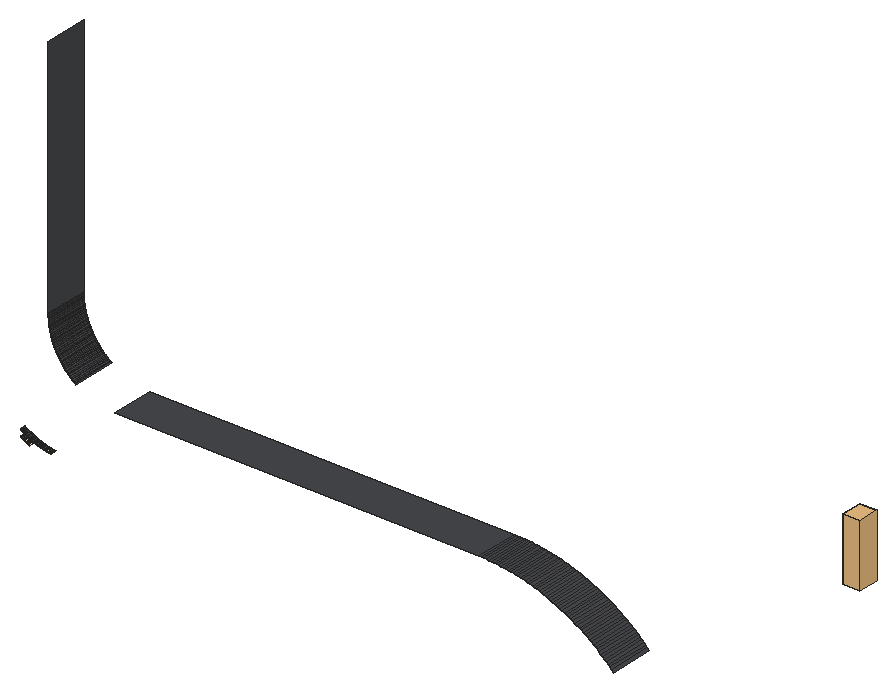
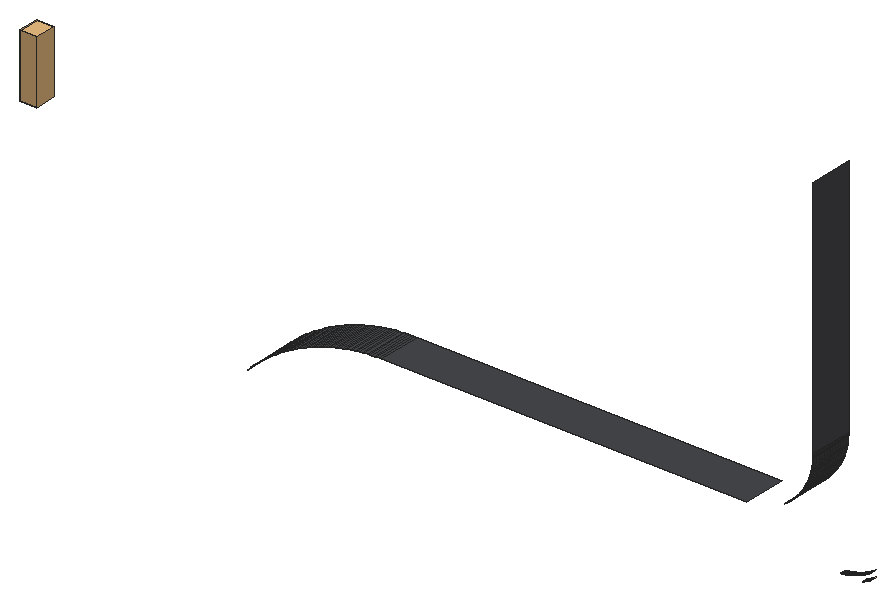
# SketchUp Ruby script. Lengths in inches.
U = 1.inch
M = Sketchup.active_model
def pt(a) = Geom::Point3d.new(a.map { |v| v * U })
def face(e, loops, mat)
  f = e.add_face(loops[0].map { |a| pt(a) })
  loops[1..].each { |l| e.add_face(l.map { |a| pt(a) }).erase! }
  f.material = f.back_material = mat if mat
  f
end
# faces: each face lists its corners as indices into pts; further lists are holes
def faces(e, pts, list, mat = nil) = list.each { |f| face(e, (f[0].is_a?(Array) ? f : [f]).map { |l| l.map { |i| pts[i] } }, mat) }
# xy, xz, yz: faces in a plane at the given z, y or x. An outline is a flat list of corners, or four numbers for a rectangle; further outlines are holes
def ring(l) = l.size == 4 ? [[l[0], l[1]], [l[2], l[1]], [l[2], l[3]], [l[0], l[3]]] : l.each_slice(2).to_a
def flat(e, list, mat, &to3) = list.each { |f| face(e, (f[0].is_a?(Array) ? f : [f]).map { |l| ring(l).map { |u, v| to3.(u, v) } }, mat) }
def xy(e, z, list, mat = nil) = flat(e, list, mat) { |x, y| [x, y, z] }
def xz(e, y, list, mat = nil) = flat(e, list, mat) { |x, z| [x, y, z] }
def yz(e, x, list, mat = nil) = flat(e, list, mat) { |y, z| [x, y, z] }
def lines(e, pts, list) = list.each { |a, b| e.add_line(pt(pts[a]), pt(pts[b])) }
# prism: a flat outline (further loops are holes) pulled along v
def prism(e, loops, v, mat = nil)
  f = face(e, loops, mat); d = Geom::Vector3d.new(v.map { |x| x * U })
  f.pushpull(f.normal.samedirection?(d) ? d.length : -d.length)
end
def box(e, o, s, mat = nil) = prism(e, [[o, [o[0] + s[0], o[1], o[2]], [o[0] + s[0], o[1] + s[1], o[2]], [o[0], o[1] + s[1], o[2]]]], [0, 0, s[2]], mat)
def at(x, y, z, deg = 0) = Geom::Transformation.translation(pt([x, y, z])) * Geom::Transformation.rotation(ORIGIN, Z_AXIS, deg.degrees)
def axes(o, x, y, z) = Geom::Transformation.new([*x, 0, *y, 0, *z, 0, *pt(o).to_a, 1])
def part(name) = M.definitions.add(name)
# library, detail: a bought-in or finely detailed component or shape, given as its bounding box
def library(name, o, s) = part(name).tap { |d| box(d.entities, o, s) }
def detail(e, o, s) = box(e.add_group.entities, o, s)
def put(e, d, t, mat = nil) = e.add_instance(d, t).tap { |i| i.material = mat if mat }
def group(e, t, mat = nil) = e.add_group.tap { |g| g.transformation = t; g.material = mat if mat }.entities
root = M.entities
M.materials.add("1432 AP 8245 TAR ROAD").color = [71, 72, 75]
M.materials.add("Outer Light").color = [251, 217, 152]
c1 = library("WALL LIGHT 69",[4.19,4.05,-8.78],[4.61,5.7,17.13])
xy(root,461.79,[[294,95.37,393,107.37],[393,95.37,393.67,107.37]],"1432 AP 8245 TAR ROAD")
yz(root,276,[[95.37,479.56,107.37,479.79],[95.37,479.79,107.37,545.79]],"1432 AP 8245 TAR ROAD")
yz(root,276.01,[[95.37,479.09,107.37,479.32]],"1432 AP 8245 TAR ROAD")
p = [[270.86,96.87,445.98],[271.01,96.87,445.91],[271.01,95.37,445.91],[270.86,95.37,445.98],[270.86,95.37,445.98],[271.01,95.37,445.91],
  [271.01,96.87,445.91],[270.86,96.87,445.98],[276.62,95.37,445.94],[276.47,95.37,445.96],[276.47,96.87,445.96],[276.62,96.87,445.94],
  [276.62,96.87,445.94],[276.47,96.87,445.96],[276.47,95.37,445.96],[276.62,95.37,445.94],[276.77,95.37,445.92],[276.77,96.87,445.92],
  [276.77,96.87,445.92],[276.77,95.37,445.92],[276.92,95.37,445.91],[276.92,96.87,445.91],[276.92,96.87,445.91],[276.92,95.37,445.91],
  [270.5625,96.87,446.11],[270.71,96.87,446.04],[270.71,95.37,446.04],[270.5625,95.37,446.11],[270.5625,95.37,446.11],[270.71,95.37,446.04],
  [270.71,96.87,446.04],[270.5625,96.87,446.11],[275.88,95.37,446.05],[275.73,95.37,446.07],[275.73,96.87,446.07],[275.88,96.87,446.05],
  [275.88,96.87,446.05],[275.73,96.87,446.07],[275.73,95.37,446.07],[275.88,95.37,446.05],[276.03,95.37,446.03],[276.03,96.87,446.03],
  [276.03,96.87,446.03],[276.03,95.37,446.03],[276.18,95.37,446],[276.18,96.87,446],[276.18,96.87,446],[276.18,95.37,446],
  [276.32,95.37,445.98],[276.32,96.87,445.98],[276.32,96.87,445.98],[276.32,95.37,445.98],[270.42,96.87,446.18],[270.42,95.37,446.18],
  [270.42,95.37,446.18],[270.42,96.87,446.18],[275.44,95.37,446.13],[275.29,95.37,446.16],[275.29,96.87,446.16],[275.44,96.87,446.13],
  [275.44,96.87,446.13],[275.29,96.87,446.16],[275.29,95.37,446.16],[275.44,95.37,446.13],[275.59,95.37,446.1],[275.59,96.87,446.1],
  [275.59,96.87,446.1],[275.59,95.37,446.1],[270.125,96.87,446.3125],[270.27,96.87,446.24],[270.27,95.37,446.24],[270.125,95.37,446.3125],
  [270.125,95.37,446.3125],[270.27,95.37,446.24],[270.27,96.87,446.24],[270.125,96.87,446.3125],[274.86,95.37,446.25],[274.71,95.37,446.28],
  [274.71,96.87,446.28],[274.86,96.87,446.25],[274.86,96.87,446.25],[274.71,96.87,446.28],[274.71,95.37,446.28],[274.86,95.37,446.25],
  [275,95.37,446.22],[275,96.87,446.22],[275,96.87,446.22],[275,95.37,446.22],[275.15,95.37,446.1875],[275.15,96.87,446.1875],
  [275.15,96.87,446.1875],[275.15,95.37,446.1875],[269.98,96.87,446.38],[269.98,95.37,446.38],[269.98,95.37,446.38],[269.98,96.87,446.38],
  [274.56,95.37,446.32],[274.42,95.37,446.35],[274.42,96.87,446.35],[274.56,96.87,446.32],[274.56,96.87,446.32],[274.42,96.87,446.35],
  [274.42,95.37,446.35],[274.56,95.37,446.32],[269.84,96.87,446.45],[269.84,95.37,446.45],[269.84,95.37,446.45],[269.84,96.87,446.45],
  [274.13,95.37,446.43],[273.99,95.37,446.47],[273.99,96.87,446.47],[274.13,96.87,446.43],[274.13,96.87,446.43],[273.99,96.87,446.47],
  [273.99,95.37,446.47],[274.13,95.37,446.43],[274.27,95.37,446.39],[274.27,96.87,446.39],[274.27,96.87,446.39],[274.27,95.37,446.39],
  [429.53,107.37,446.38],[429.0625,107.37,446.85],[429.0625,95.37,446.85],[429.53,95.37,446.38],[269.55,96.87,446.6],[269.69,96.87,446.53],
  [269.69,95.37,446.53],[269.55,95.37,446.6],[269.55,95.37,446.6],[269.69,95.37,446.53],[269.69,96.87,446.53],[269.55,96.87,446.6],
  [273.7,95.37,446.55],[273.56,95.37,446.59],[273.56,96.87,446.59],[273.7,96.87,446.55],[273.7,96.87,446.55],[273.56,96.87,446.59],
  [273.56,95.37,446.59],[273.7,95.37,446.55],[273.84,95.37,446.51],[273.84,96.87,446.51],[273.84,96.87,446.51],[273.84,95.37,446.51],
  [269.41,96.87,446.67],[269.41,95.37,446.67],[269.41,95.37,446.67],[269.41,96.87,446.67],[273.41,95.37,446.63],[273.27,95.37,446.68],
  [273.27,96.87,446.68],[273.41,96.87,446.63],[273.41,96.87,446.63],[273.27,96.87,446.68],[273.27,95.37,446.68],[273.41,95.37,446.63],
  [269.27,96.87,446.75],[269.27,95.37,446.75],[269.27,95.37,446.75],[269.27,96.87,446.75],[273.13,95.37,446.72],[272.99,95.37,446.77],
  [272.99,96.87,446.77],[273.13,96.87,446.72],[273.13,96.87,446.72],[272.99,96.87,446.77],[272.99,95.37,446.77],[273.13,95.37,446.72],
  [268.98,96.87,446.91],[269.125,96.87,446.83],[269.125,95.37,446.83],[268.98,95.37,446.91],[268.98,95.37,446.91],[269.125,95.37,446.83],
  [269.125,96.87,446.83],[268.98,96.87,446.91],[272.85,95.37,446.82],[272.7,95.37,446.87],[272.7,96.87,446.87],[272.85,96.87,446.82],
  [272.85,96.87,446.82],[272.7,96.87,446.87],[272.7,95.37,446.87],[272.85,95.37,446.82],[268.84,96.87,446.99],[268.84,95.37,446.99],
  [268.84,95.37,446.99],[268.84,96.87,446.99],[272.5625,95.37,446.92],[272.42,95.37,446.97],[272.42,96.87,446.97],[272.5625,96.87,446.92],
  [272.5625,96.87,446.92],[272.42,96.87,446.97],[272.42,95.37,446.97],[272.5625,95.37,446.92],[428.59,107.37,447.32],[428.59,95.37,447.32],
  [268.7,96.87,447.07],[268.7,95.37,447.07],[268.7,95.37,447.07],[268.7,96.87,447.07],[272.28,95.37,447.02],[272.14,95.37,447.07],
  [272.14,96.87,447.07],[272.28,96.87,447.02],[272.28,96.87,447.02],[272.14,96.87,447.07],[272.14,95.37,447.07],[272.28,95.37,447.02],
  [268.43,96.87,447.23],[268.56,96.87,447.15],[268.56,95.37,447.15],[268.43,95.37,447.23],[268.56,95.37,447.15],[268.56,96.87,447.15],
  [272.01,95.37,447.125],[271.87,95.37,447.18],[271.87,96.87,447.18],[272.01,96.87,447.125],[272.01,96.87,447.125],[271.87,96.87,447.18],
  [271.87,95.37,447.18],[272.01,95.37,447.125],[271.73,95.37,447.24],[271.59,95.37,447.3],[271.59,96.87,447.3],[271.73,96.87,447.24],
  [271.73,96.87,447.24],[271.59,96.87,447.3],[271.59,95.37,447.3],[271.73,95.37,447.24],[271.45,95.37,447.35],[271.45,96.87,447.35],
  [271.45,96.87,447.35],[271.45,95.37,447.35],[428.11,107.37,447.79],[428.11,95.37,447.79],[271.32,95.37,447.41],[271.18,95.37,447.48],
  [271.18,96.87,447.48],[271.32,96.87,447.41],[271.32,96.87,447.41],[271.18,96.87,447.48],[271.18,95.37,447.48],[271.32,95.37,447.41],
  [271.05,95.37,447.54],[270.91,95.37,447.6],[270.91,96.87,447.6],[271.05,96.87,447.54],[271.05,96.87,447.54],[270.91,96.87,447.6],
  [270.91,95.37,447.6],[271.05,95.37,447.54],[270.78,95.37,447.66],[270.78,96.87,447.66],[270.78,96.87,447.66],[270.78,95.37,447.66],
  [270.64,95.37,447.73],[270.51,95.37,447.8],[270.51,96.87,447.8],[270.64,96.87,447.73],[270.64,96.87,447.73],[270.51,96.87,447.8],
  [270.51,95.37,447.8],[270.64,95.37,447.73],[270.375,95.37,447.86],[270.375,96.87,447.86],[270.375,96.87,447.86],[270.375,95.37,447.86],
  [427.62,107.37,448.24],[427.62,95.37,448.24],[270.24,95.37,447.93],[270.11,95.37,448],[270.11,96.87,448],[270.24,96.87,447.93],
  [270.24,96.87,447.93],[270.11,96.87,448],[270.11,95.37,448],[270.24,95.37,447.93],[269.98,95.37,448.07],[269.98,96.87,448.07],
  [269.98,96.87,448.07],[269.98,95.37,448.07],[269.85,95.37,448.14],[269.72,95.37,448.21],[269.72,96.87,448.21],[269.85,96.87,448.14],
  [269.85,96.87,448.14],[269.72,96.87,448.21],[269.72,95.37,448.21],[269.85,95.37,448.14],[269.59,95.37,448.29],[269.59,96.87,448.29],
  [269.59,96.87,448.29],[269.59,95.37,448.29],[427.125,107.37,448.69],[427.125,95.37,448.69],[269.46,95.37,448.36],[269.46,96.87,448.36],
  [269.46,96.87,448.36],[269.46,95.37,448.36],[269.33,95.37,448.4375],[269.2,95.37,448.51],[269.2,96.87,448.51],[269.33,96.87,448.4375],
  [269.33,96.87,448.4375],[269.2,96.87,448.51],[269.2,95.37,448.51],[269.33,95.37,448.4375],[269.07,95.37,448.59],[269.07,96.87,448.59],
  [269.07,96.87,448.59],[269.07,95.37,448.59],[268.95,95.37,448.67],[268.95,96.87,448.67],[268.95,96.87,448.67],[268.95,95.37,448.67],
  [268.82,95.37,448.75],[268.69,95.37,448.83],[268.69,96.87,448.83],[268.82,96.87,448.75],[268.82,96.87,448.75],[268.69,96.87,448.83],
  [268.69,95.37,448.83],[268.82,95.37,448.75],[426.625,107.37,449.14],[426.625,95.37,449.14],[268.57,95.37,448.91],[268.57,96.87,448.91],
  [268.57,96.87,448.91],[268.57,95.37,448.91],[268.44,95.37,448.99],[268.44,96.87,448.99],[268.44,96.87,448.99],[268.44,95.37,448.99],
  [426.12,107.37,449.57],[426.12,95.37,449.57],[425.61,107.37,450],[425.61,95.37,450],[425.1,107.37,450.43],[425.1,95.37,450.43],
  [424.57,107.37,450.84],[424.57,95.37,450.84],[424.05,107.37,451.25],[424.05,95.37,451.25],[423.51,107.37,451.66],[423.51,95.37,451.66],
  [422.98,107.37,452.05],[422.98,95.37,452.05],[422.43,107.37,452.44],[422.43,95.37,452.44],[421.89,107.37,452.82],[421.89,95.37,452.82],
  [421.33,107.37,453.2],[421.33,95.37,453.2],[420.78,107.37,453.5625],[420.78,95.37,453.5625],[420.21,107.37,453.92],[420.21,95.37,453.92],
  [419.65,107.37,454.28],[419.65,95.37,454.28],[419.08,107.37,454.62],[419.08,95.37,454.62],[418.5,107.37,454.96],[418.5,95.37,454.96],
  [417.92,107.37,455.29],[417.92,95.37,455.29],[417.34,107.37,455.61],[417.34,95.37,455.61],[416.75,107.37,455.93],[416.75,95.37,455.93],
  [416.15,107.37,456.23],[416.15,95.37,456.23],[415.56,107.37,456.53],[415.56,95.37,456.53],[414.96,107.37,456.82],[414.96,95.37,456.82],
  [414.35,107.37,457.11],[414.35,95.37,457.11],[413.74,107.37,457.38],[413.74,95.37,457.38],[413.13,107.37,457.65],[413.13,95.37,457.65],
  [412.52,107.37,457.91],[412.52,95.37,457.91],[411.9,107.37,458.16],[411.9,95.37,458.16],[411.28,107.37,458.4],[411.28,95.37,458.4],
  [410.65,107.37,458.64],[410.65,95.37,458.64],[410.02,107.37,458.87],[410.02,95.37,458.87],[409.39,107.37,459.09],[409.39,95.37,459.09],
  [408.76,107.37,459.3],[408.76,95.37,459.3],[408.125,107.37,459.5],[408.125,95.37,459.5],[407.48,107.37,459.69],[407.48,95.37,459.69],
  [406.84,107.37,459.88],[406.84,95.37,459.88],[406.2,107.37,460.05],[406.2,95.37,460.05],[405.55,107.37,460.22],[405.55,95.37,460.22],
  [404.91,107.37,460.38],[404.91,95.37,460.38],[404.26,107.37,460.53],[404.26,95.37,460.53],[403.6,107.37,460.68],[403.6,95.37,460.68],
  [402.95,107.37,460.8125],[402.95,95.37,460.8125],[402.29,107.37,460.9375],[402.29,95.37,460.9375],[401.64,107.37,461.06],[401.64,95.37,461.06],
  [400.98,107.37,461.16],[400.98,95.37,461.16],[400.32,107.37,461.26],[400.32,95.37,461.26],[399.66,107.37,461.36],[399.66,95.37,461.36],
  [398.99,107.37,461.4375],[398.33,107.37,461.51],[398.33,95.37,461.51],[398.99,95.37,461.4375],[397.67,107.37,461.58],[397.67,95.37,461.58],
  [397,107.37,461.63],[396.34,107.37,461.68],[396.34,95.37,461.68],[397,95.37,461.63],[395.67,107.37,461.72],[395,107.37,461.75],
  [395,95.37,461.75],[395.67,95.37,461.72],[394.34,107.37,461.77],[393.67,107.37,461.79],[393.67,95.37,461.79],[394.34,95.37,461.77],
  [283.61,107.37,465.09],[283.42,107.37,465.23],[283.42,95.37,465.23],[283.61,95.37,465.09],[283.23,107.37,465.37],[283.23,95.37,465.37],
  [283.04,107.37,465.51],[283.04,95.37,465.51],[282.86,107.37,465.66],[282.86,95.37,465.66],[282.67,107.37,465.8],[282.67,95.37,465.8],
  [282.49,107.37,465.95],[282.49,95.37,465.95],[282.31,107.37,466.1],[282.31,95.37,466.1],[282.13,107.37,466.26],[282.13,95.37,466.26],
  [281.96,107.37,466.42],[281.96,95.37,466.42],[281.78,107.37,466.57],[281.78,95.37,466.57],[281.61,107.37,466.74],[281.61,95.37,466.74],
  [281.44,107.37,466.9],[281.44,95.37,466.9],[281.27,107.37,467.0625],[281.27,95.37,467.0625],[281.11,107.37,467.23],[281.11,95.37,467.23],
  [280.94,107.37,467.4],[280.94,95.37,467.4],[280.78,107.37,467.57],[280.78,95.37,467.57],[280.625,107.37,467.75],[280.625,95.37,467.75],
  [280.47,107.37,467.92],[280.47,95.37,467.92],[280.3125,107.37,468.1],[280.3125,95.37,468.1],[280.16,107.37,468.28],[280.16,95.37,468.28],
  [280.01,107.37,468.46],[280.01,95.37,468.46],[279.86,107.37,468.65],[279.86,95.37,468.65],[279.72,107.37,468.83],[279.72,95.37,468.83],
  [279.58,107.37,469.02],[279.58,95.37,469.02],[279.4375,107.37,469.21],[279.4375,95.37,469.21],[279.3,107.37,469.4],[279.3,95.37,469.4],
  [279.17,107.37,469.6],[279.17,95.37,469.6],[279.03,107.37,469.79],[279.03,95.37,469.79],[278.9,107.37,469.99],[278.9,95.37,469.99],
  [278.78,107.37,470.1875],[278.78,95.37,470.1875],[278.65,107.37,470.39],[278.65,95.37,470.39],[278.53,107.37,470.59],[278.53,95.37,470.59],
  [278.41,107.37,470.79],[278.41,95.37,470.79],[278.3,107.37,471],[278.3,95.37,471],[278.18,107.37,471.2],[278.18,95.37,471.2],
  [278.07,107.37,471.41],[278.07,95.37,471.41],[277.96,107.37,471.62],[277.96,95.37,471.62],[277.86,107.37,471.83],[277.86,95.37,471.83],
  [277.75,107.37,472.04],[277.75,95.37,472.04],[277.65,107.37,472.26],[277.65,95.37,472.26],[277.56,107.37,472.47],[277.56,95.37,472.47],
  [277.46,107.37,472.6875],[277.46,95.37,472.6875],[277.37,107.37,472.9],[277.37,95.37,472.9],[277.28,107.37,473.12],[277.28,95.37,473.12],
  [277.2,107.37,473.34],[277.2,95.37,473.34],[277.11,107.37,473.5625],[277.11,95.37,473.5625],[277.03,107.37,473.78],[277.03,95.37,473.78],
  [276.96,107.37,474.01],[276.96,95.37,474.01],[276.88,107.37,474.23],[276.88,95.37,474.23],[276.81,107.37,474.45],[276.81,95.37,474.45],
  [276.74,107.37,474.68],[276.74,95.37,474.68],[276.68,107.37,474.91],[276.68,95.37,474.91],[276.61,107.37,475.13],[276.61,95.37,475.13],
  [276.55,107.37,475.36],[276.55,95.37,475.36],[276.5,107.37,475.59],[276.5,95.37,475.59],[276.44,107.37,475.82],[276.44,95.37,475.82],
  [276.39,107.37,476.05],[276.39,95.37,476.05],[276.35,107.37,476.28],[276.35,95.37,476.28],[276.3,107.37,476.51],[276.3,95.37,476.51],
  [276.26,107.37,476.74],[276.26,95.37,476.74],[276.22,107.37,476.98],[276.22,95.37,476.98],[276.1875,107.37,477.21],[276.1875,95.37,477.21],
  [276.15,107.37,477.44],[276.15,95.37,477.44],[276.125,107.37,477.68],[276.125,95.37,477.68],[276.1,107.37,477.91],[276.1,95.37,477.91],
  [276.08,107.37,478.15],[276.08,95.37,478.15],[276.06,107.37,478.38],[276.06,95.37,478.38],[276.04,107.37,478.61],[276.04,95.37,478.61],
  [276.02,107.37,478.85],[276.02,95.37,478.85],[276.01,107.37,479.09],[276.01,95.37,479.09],[276.01,107.37,479.32],[276,107.37,479.56],
  [276,95.37,479.56],[276.01,95.37,479.32]]
faces(root,p,[[0,1,2,3],[12,13,14,15],[18,12,15,19],[22,18,19,23],[24,25,26,27],[25,0,3,26],[36,37,38,39],[42,36,39,43],
  [46,42,43,47],[50,46,47,51],[13,50,51,14],[52,24,27,53],[60,61,62,63],[66,60,63,67],[37,66,67,38],[68,69,70,71],
  [69,52,53,70],[80,81,82,83],[86,80,83,87],[90,86,87,91],[61,90,91,62],[92,68,71,93],[100,101,102,103],[81,100,103,82],
  [104,92,93,105],[112,113,114,115],[118,112,115,119],[101,118,119,102],[124,125,126,127],[125,104,105,126],[136,137,138,139],[142,136,139,143],
  [113,142,143,114],[144,124,127,145],[152,153,154,155],[137,152,155,138],[156,144,145,157],[164,165,166,167],[153,164,167,154],[168,169,170,171],
  [169,156,157,170],[180,181,182,183],[165,180,183,166],[184,168,171,185],[192,193,194,195],[181,192,195,182],[198,184,185,199],[206,207,208,209],
  [193,206,209,194],[210,211,212,213],[211,198,199,212],[220,221,222,223],[207,220,223,208],[228,229,230,231],[221,228,231,222],[229,234,235,230],
  [242,243,244,245],[234,242,245,235],[250,251,252,253],[243,250,253,244],[251,256,257,252],[262,263,264,265],[256,262,265,257],[263,268,269,264],
  [276,277,278,279],[268,276,279,269],[277,282,283,278],[288,289,290,291],[282,288,291,283],[289,294,295,290],[294,300,301,295],[306,307,308,309],
  [300,306,309,301],[307,312,313,308],[312,316,317,313],[322,323,324,325],[316,322,325,317],[323,330,331,324],[330,334,335,331]],"Outer Light")
faces(root,p,[[4,5,6,7],[8,9,10,11],[16,8,11,17],[20,16,17,21],[28,29,30,31],[29,4,7,30],[32,33,34,35],[40,32,35,41],
  [44,40,41,45],[48,44,45,49],[9,48,49,10],[54,28,31,55],[56,57,58,59],[64,56,59,65],[33,64,65,34],[72,73,74,75],
  [73,54,55,74],[76,77,78,79],[84,76,79,85],[88,84,85,89],[57,88,89,58],[94,72,75,95],[96,97,98,99],[77,96,99,78],
  [106,94,95,107],[108,109,110,111],[116,108,111,117],[97,116,117,98],[120,121,122,123],[128,129,130,131],[129,106,107,130],[132,133,134,135],
  [140,132,135,141],[109,140,141,110],[146,128,131,147],[148,149,150,151],[133,148,151,134],[158,146,147,159],[160,161,162,163],[149,160,163,150],
  [172,173,174,175],[173,158,159,174],[176,177,178,179],[161,176,179,162],[186,172,175,187],[188,189,190,191],[177,188,191,178],[121,196,197,122],
  [200,186,187,201],[202,203,204,205],[189,202,205,190],[214,200,201,215],[216,217,218,219],[203,216,219,204],[224,225,226,227],[217,224,227,218],
  [225,232,233,226],[196,236,237,197],[238,239,240,241],[232,238,241,233],[246,247,248,249],[239,246,249,240],[247,254,255,248],[258,259,260,261],
  [254,258,261,255],[259,266,267,260],[236,270,271,237],[272,273,274,275],[266,272,275,267],[273,280,281,274],[284,285,286,287],[280,284,287,281],
  [285,292,293,286],[270,296,297,271],[292,298,299,293],[302,303,304,305],[298,302,305,299],[303,310,311,304],[310,314,315,311],[318,319,320,321],
  [314,318,321,315],[296,326,327,297],[319,328,329,320],[328,332,333,329],[326,336,337,327],[336,338,339,337],[338,340,341,339],[340,342,343,341],
  [342,344,345,343],[344,346,347,345],[346,348,349,347],[348,350,351,349],[350,352,353,351],[352,354,355,353],[354,356,357,355],[356,358,359,357],
  [358,360,361,359],[360,362,363,361],[362,364,365,363],[364,366,367,365],[366,368,369,367],[368,370,371,369],[370,372,373,371],[372,374,375,373],
  [374,376,377,375],[376,378,379,377],[378,380,381,379],[380,382,383,381],[382,384,385,383],[384,386,387,385],[386,388,389,387],[388,390,391,389],
  [390,392,393,391],[392,394,395,393],[394,396,397,395],[396,398,399,397],[398,400,401,399],[400,402,403,401],[402,404,405,403],[404,406,407,405],
  [406,408,409,407],[408,410,411,409],[410,412,413,411],[412,414,415,413],[414,416,417,415],[416,418,419,417],[418,420,421,419],[420,422,423,421],
  [422,424,425,423],[426,427,428,429],[424,426,429,425],[427,430,431,428],[432,433,434,435],[430,432,435,431],[436,437,438,439],[433,436,439,434],
  [440,441,442,443],[437,440,443,438],[444,445,446,447],[445,448,449,446],[448,450,451,449],[450,452,453,451],[452,454,455,453],[454,456,457,455],
  [456,458,459,457],[458,460,461,459],[460,462,463,461],[462,464,465,463],[464,466,467,465],[466,468,469,467],[468,470,471,469],[470,472,473,471],
  [472,474,475,473],[474,476,477,475],[476,478,479,477],[478,480,481,479],[480,482,483,481],[482,484,485,483],[484,486,487,485],[486,488,489,487],
  [488,490,491,489],[490,492,493,491],[492,494,495,493],[494,496,497,495],[496,498,499,497],[498,500,501,499],[500,502,503,501],[502,504,505,503],
  [504,506,507,505],[506,508,509,507],[508,510,511,509],[510,512,513,511],[512,514,515,513],[514,516,517,515],[516,518,519,517],[518,520,521,519],
  [520,522,523,521],[522,524,525,523],[524,526,527,525],[526,528,529,527],[528,530,531,529],[530,532,533,531],[532,534,535,533],[534,536,537,535],
  [536,538,539,537],[538,540,541,539],[540,542,543,541],[542,544,545,543],[544,546,547,545],[546,548,549,547],[548,550,551,549],[550,552,553,551],
  [552,554,555,553],[554,556,557,555],[556,558,559,557],[558,560,561,559],[560,562,563,561],[562,564,565,563],[564,566,567,565],[566,568,569,567],
  [568,570,571,569],[570,572,573,571],[572,574,575,573],[574,576,577,575],[576,578,579,577],[578,580,581,579],[580,582,583,581],[582,584,585,583],
  [586,587,588,589]],"1432 AP 8245 TAR ROAD")
put(root,c1,at(485.24,94.12,496.41))
